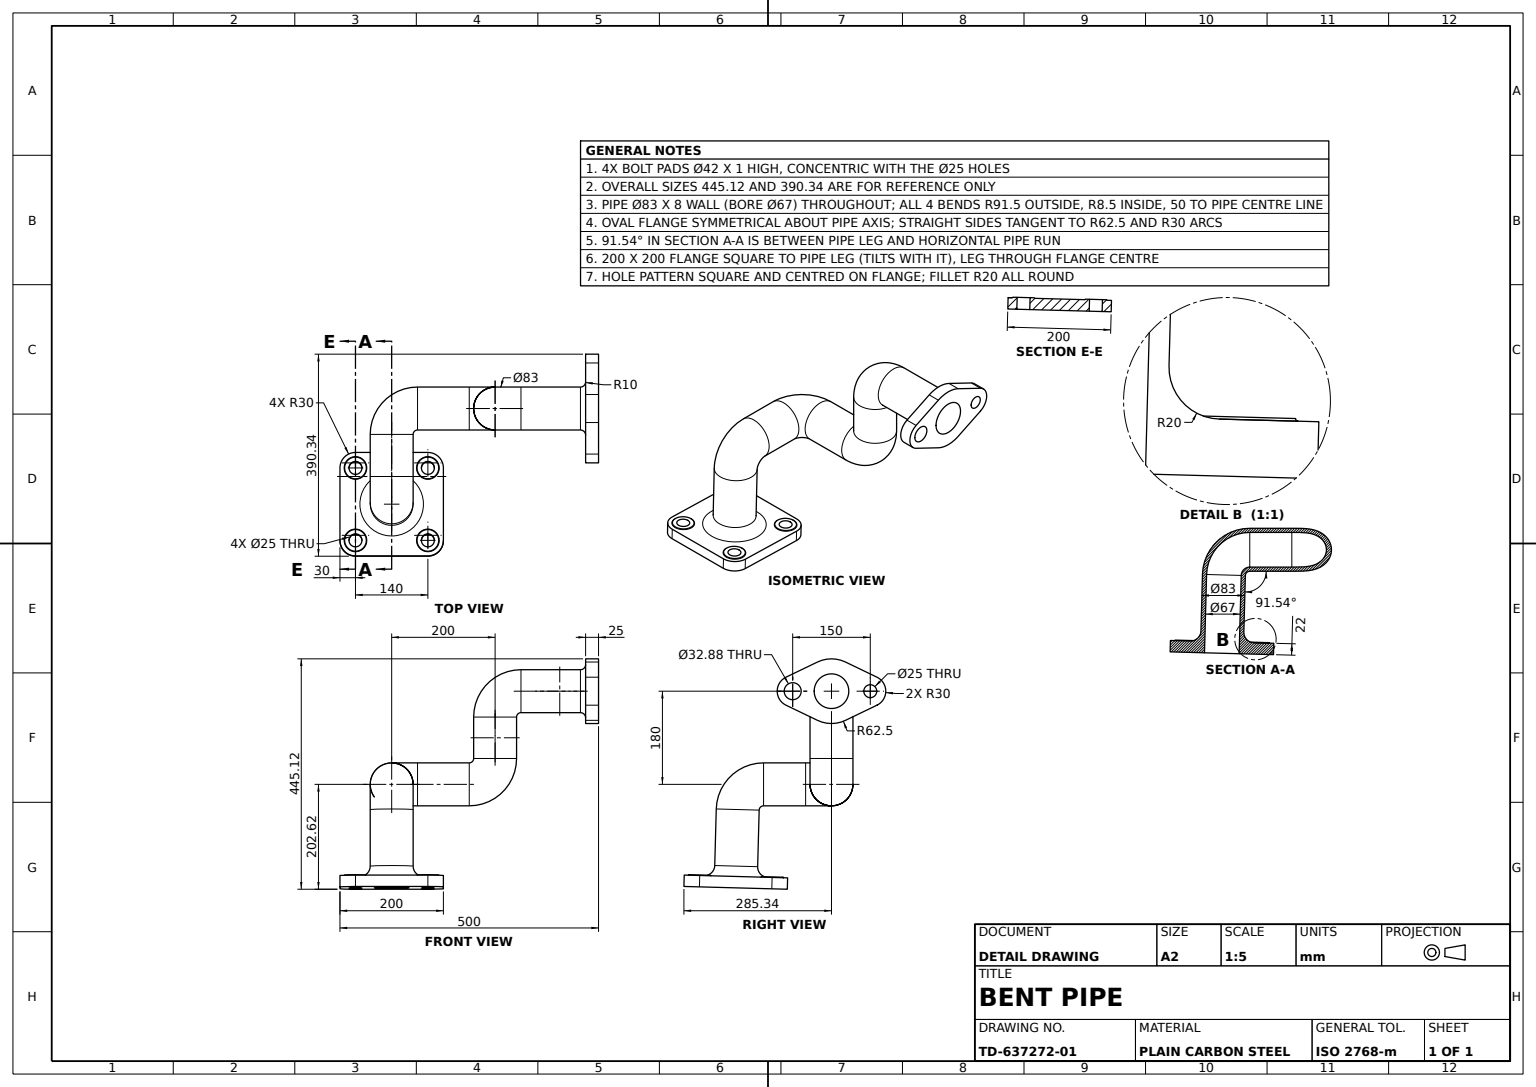
solid
v1 (0,0,-105)
v2 (0,27.037012,-88)
e1 v1 v2 CIRCLE(AX(P(0,0,-75),D(1,0,0),D(0,0,-1)),30)
v3 (-25,0,-105)
e2 v3 v1 LINE
v4 (-25,27.037012,-88)
e3 v3 v4 CIRCLE(AX(P(-25,0,-75),D(1,0,0),D(0,0,-1)),30)
e4 v4 v2 LINE
face CYL(AX(P(-25,0,-75),D(1,0,0),D(0,0,-1)),30) [-e1 -e2 e3 e4]
v5 (-25,0,-62.5)
v6 (-25,0,-87.5)
e5 v5 v6 CIRCLE(AX(P(-25,0,-75),D(1,0,0),D(0,0,-1)),12.5)
e6 v6 v5 CIRCLE(AX(P(-25,0,-75),D(1,0,0),D(0,0,-1)),12.5)
v7 (-25,27.037012,88)
v8 (-25,-27.037012,88)
e7 v7 v8 CIRCLE(AX(P(-25,0,75),D(1,0,0),D(0,0,-1)),30)
v9 (-25,56.327108,27.083333)
e8 v9 v7 LINE
v10 (-25,56.327108,-27.083333)
e9 v10 v9 CIRCLE(AX(P(-25,0,0),D(1,0,0),D(0,0,-1)),62.5)
e10 v4 v10 LINE
v11 (-25,-27.037012,-88)
e11 v11 v3 CIRCLE(AX(P(-25,0,-75),D(1,0,0),D(0,0,-1)),30)
v12 (-25,-56.327108,-27.083333)
e12 v12 v11 LINE
v13 (-25,-56.327108,27.083333)
e13 v13 v12 CIRCLE(AX(P(-25,0,0),D(1,0,0),D(0,0,-1)),62.5)
e14 v8 v13 LINE
v14 (-25,0,-51.5)
v15 (-25,0,51.5)
e15 v14 v15 CIRCLE(AX(P(-25,0,0),D(1,0,0),D(0,0,-1)),51.5)
e16 v15 v14 CIRCLE(AX(P(-25,0,0),D(1,0,0),D(0,0,-1)),51.5)
v16 (-25,0,91.441402)
v17 (-25,0,58.558598)
e17 v16 v17 CIRCLE(AX(P(-25,0,75),D(1,0,0),D(0,0,-1)),16.441402)
e18 v17 v16 CIRCLE(AX(P(-25,0,75),D(1,0,0),D(0,0,-1)),16.441402)
face PLANE(AX(P(-25,0,75),D(1,0,0),D(0,0,-1))) rev [e5 e6] [-e7 -e8 -e9 -e10 -e3 -e11 -e12 -e13 -e14] [e15 e16] [e17 e18]
v18 (0,-27.037012,88)
e19 v8 v18 LINE
v19 (0,27.037012,88)
e20 v19 v18 CIRCLE(AX(P(0,0,75),D(1,0,0),D(0,0,-1)),30)
e21 v7 v19 LINE
face CYL(AX(P(-25,0,75),D(1,0,0),D(0,0,-1)),30) [e7 e19 -e20 -e21]
v20 (-330,-355.247197,284.74932)
v21 (-330,-377.239245,285.340782)
e22 v20 v21 LINE
v22 (-300,-378.045784,255.351625)
e23 v22 v21 CIRCLE(AX(P(-330,-378.045784,255.351625),D(0,-0.999638543,0.026884636),D(0,-0.026884636,-0.999638543)),30)
v23 (-300,-356.053736,254.760163)
e24 v23 v22 LINE
e25 v23 v20 CIRCLE(AX(P(-330,-356.053736,254.760163),D(0,-0.999638543,0.026884636),D(0,-0.026884636,-0.999638543)),30)
face CYL(AX(P(-330,-356.053736,254.760163),D(0,-0.999638543,0.026884636),D(0,-0.026884636,-0.999638543)),30) [e22 -e23 -e24 e25]
v24 (0,-56.327108,27.083333)
e26 v13 v24 LINE
v25 (0,-56.327108,-27.083333)
e27 v12 v25 LINE
e28 v24 v25 CIRCLE(AX(P(0,0,0),D(1,0,0),D(0,0,-1)),62.5)
face CYL(AX(P(-25,0,0),D(1,0,0),D(0,0,-1)),62.5) [-e26 e13 e27 -e28]
v26 (-200,-50,-33.5)
v27 (-200,-130,-33.5)
e29 v26 v27 LINE
v28 (-233.5,-50,0)
e30 v26 v28 CIRCLE(AX(P(-200,-50,0),D(0,1,0),D(-1,0,0)),33.5)
v29 (-200,-50,33.5)
e31 v28 v29 CIRCLE(AX(P(-200,-50,0),D(0,1,0),D(-1,0,0)),33.5)
v30 (-200,-130,33.5)
e32 v29 v30 LINE
v31 (-233.5,-130,0)
e33 v31 v30 CIRCLE(AX(P(-200,-130,0),D(0,1,0),D(0,0,-1)),33.5)
e34 v27 v31 CIRCLE(AX(P(-200,-130,0),D(0,1,0),D(0,0,-1)),33.5)
face CYL(AX(P(-200,-50,0),D(0,-1,0),D(0,0,-1)),33.5) rev [-e29 e30 e31 e32 -e33 -e34]
v32 (-500,-359.817585,114.810767)
v33 (-500,-381.809633,115.402229)
e35 v32 v33 LINE
v34 (-470,-360.624124,84.821611)
e36 v32 v34 CIRCLE(AX(P(-470,-359.817585,114.810767),D(0,-0.999638543,0.026884636),D(0,-0.026884636,-0.999638543)),30)
v35 (-470,-382.616172,85.413073)
e37 v34 v35 LINE
e38 v33 v35 CIRCLE(AX(P(-470,-381.809633,115.402229),D(0,-0.999638543,0.026884636),D(0,-0.026884636,-0.999638543)),30)
face CYL(AX(P(-470,-359.817585,114.810767),D(0,-0.999638543,0.026884636),D(0,-0.026884636,-0.999638543)),30) [-e35 e36 e37 -e38]
v36 (-470,-378.381842,242.856143)
v37 (-470,-377.709726,267.847107)
e39 v36 v37 CIRCLE(AX(P(-470,-378.045784,255.351625),D(0,-0.999638543,0.026884636),D(0,-0.026884636,-0.999638543)),12.5)
v38 (-470,-354.71804,267.22876)
e40 v38 v37 LINE
v39 (-470,-355.390155,242.237797)
e41 v38 v39 CIRCLE(AX(P(-470,-355.054098,254.733279),D(0,0.999638543,-0.026884636),D(0,0.026884636,0.999638543)),12.5)
e42 v39 v36 LINE
face CYL(AX(P(-470,-356.053736,254.760163),D(0,-0.999638543,0.026884636),D(0,-0.026884636,-0.999638543)),12.5) rev [e39 -e40 e41 e42]
v40 (-330,-381.473575,127.897711)
v41 (-330,-382.145691,102.906747)
e43 v40 v41 CIRCLE(AX(P(-330,-381.809633,115.402229),D(0,-0.999638543,0.026884636),D(0,-0.026884636,-0.999638543)),12.5)
v42 (-330,-359.154005,102.288401)
e44 v42 v41 LINE
v43 (-330,-358.481889,127.279364)
e45 v42 v43 CIRCLE(AX(P(-330,-358.817947,114.783883),D(0,0.999638543,-0.026884636),D(0,0.026884636,0.999638543)),12.5)
e46 v43 v40 LINE
face CYL(AX(P(-330,-359.817585,114.810767),D(0,-0.999638543,0.026884636),D(0,-0.026884636,-0.999638543)),12.5) rev [e43 -e44 e45 e46]
v44 (-350,-213.5,0)
v45 (-350,-180,-33.5)
e47 v44 v45 CIRCLE(AX(P(-350,-180,0),D(1,0,0),D(0,-1,0)),33.5)
v46 (-250,-213.5,0)
e48 v46 v44 LINE
v47 (-250,-146.5,0)
e49 v46 v47 CIRCLE(AX(P(-250,-180,0),D(1,0,0),D(0,1,0)),33.5)
v48 (-350,-146.5,0)
e50 v47 v48 LINE
e51 v45 v48 CIRCLE(AX(P(-350,-180,0),D(1,0,0),D(0,-1,0)),33.5)
face CYL(AX(P(-250,-180,0),D(-1,0,0),D(0,-1,0)),33.5) rev [-e47 -e48 e49 e50 -e51]
v49 (0,0,58.558598)
v50 (0,0,91.441402)
e52 v49 v50 CIRCLE(AX(P(0,0,75),D(1,0,0),D(0,0,-1)),16.441402)
e53 v16 v50 LINE
e54 v17 v49 LINE
face CYL(AX(P(-25,0,75),D(1,0,0),D(0,0,-1)),16.441402) rev [e52 -e53 -e18 e54]
v51 (-433.5,-180,50)
v52 (-366.5,-180,50)
e55 v51 v52 CIRCLE(AX(P(-400,-180,50),D(0,0,-1),D(-1,0,0)),33.5)
e56 v45 v51 CIRCLE(AX(P(-350,-180,50),D(0,1,0),D(0,0,1)),83.5)
v53 (-350,-180,33.5)
e57 v48 v53 CIRCLE(AX(P(-350,-180,0),D(1,0,0),D(0,-1,0)),33.5)
e58 v53 v52 CIRCLE(AX(P(-350,-180,50),D(0,1,0),D(0,0,1)),16.5)
face TORUS(AX(P(-350,-180,50),D(0,1,0),D(0,0,1)),50,33.5) rev [-e55 -e56 e51 e57 e58]
v54 (-500,-378.045784,255.351625)
e59 v54 v33 LINE
v55 (-500,-356.053736,254.760163)
e60 v55 v54 LINE
e61 v55 v32 LINE
face PLANE(AX(P(-500,-359.817585,114.810767),D(-1,0,0),D(0,-1,0))) [-e59 -e60 e61 e35]
v56 (-330,-355.462274,276.752211)
v57 (-330,-356.645198,232.768115)
e62 v56 v57 CIRCLE(AX(P(-330,-356.053736,254.760163),D(0,-0.999638543,0.026884636),D(0,-0.026884636,-0.999638543)),22)
v58 (-330,-354.48952,275.725688)
e63 v56 v58 CIRCLE(AX(P(-330,-354.462636,276.725327),D(1,0,0),D(0,1,0)),1)
v59 (-330,-355.618675,233.740869)
e64 v59 v58 CIRCLE(AX(P(-330,-355.054098,254.733279),D(0,0.999638543,-0.026884636),D(0,0.026884636,0.999638543)),21)
e65 v57 v59 CIRCLE(AX(P(-330,-355.64556,232.741231),D(-1,0,0),D(0,-1,0)),1)
face TORUS(AX(P(-330,-355.054098,254.733279),D(0,-0.999638543,0.026884636),D(0,-0.026884636,-0.999638543)),22,1) rev [-e62 e63 -e64 -e65]
v60 (-400,-138.5,131.326638)
v61 (-358.5,-180,131.326638)
e66 v60 v61 CIRCLE(AX(P(-400,-180,131.326638),D(0,0,-1),D(1,0,0)),41.5)
v62 (-358.5,-180,50)
e67 v62 v61 LINE
v63 (-441.5,-180,50)
e68 v63 v62 CIRCLE(AX(P(-400,-180,50),D(0,0,-1),D(-1,0,0)),41.5)
v64 (-441.5,-180,131.326638)
e69 v63 v64 LINE
e70 v64 v60 CIRCLE(AX(P(-400,-180,131.326638),D(0,0,-1),D(1,0,0)),41.5)
face CYL(AX(P(-400,-180,50),D(0,0,1),D(1,0,0)),41.5) [e66 -e67 -e68 e69 e70]
e71 v58 v59 CIRCLE(AX(P(-330,-355.054098,254.733279),D(0,0.999638543,-0.026884636),D(0,0.026884636,0.999638543)),21)
e72 v57 v56 CIRCLE(AX(P(-330,-356.053736,254.760163),D(0,-0.999638543,0.026884636),D(0,-0.026884636,-0.999638543)),22)
face TORUS(AX(P(-330,-355.054098,254.733279),D(0,-0.999638543,0.026884636),D(0,-0.026884636,-0.999638543)),22,1) rev [e65 -e71 -e63 -e72]
v65 (-150,0,41.5)
v66 (-150,-41.5,0)
e73 v65 v66 CIRCLE(AX(P(-150,0,0),D(1,0,0),D(0,0,1)),41.5)
v67 (-150,41.5,0)
e74 v67 v65 CIRCLE(AX(P(-150,0,0),D(1,0,0),D(0,0,1)),41.5)
v68 (-241.5,-50,0)
e75 v67 v68 CIRCLE(AX(P(-150,-50,0),D(0,0,1),D(0,-1,0)),91.5)
v69 (-200,-50,41.5)
e76 v68 v69 CIRCLE(AX(P(-200,-50,0),D(0,1,0),D(-1,0,0)),41.5)
v70 (-158.5,-50,0)
e77 v69 v70 CIRCLE(AX(P(-200,-50,0),D(0,1,0),D(-1,0,0)),41.5)
e78 v66 v70 CIRCLE(AX(P(-150,-50,0),D(0,0,1),D(0,-1,0)),8.5)
face TORUS(AX(P(-150,-50,0),D(0,0,1),D(0,-1,0)),50,41.5) [-e73 -e74 e75 e76 e77 -e78]
v71 (-150,-33.5,0)
v72 (-150,0,-33.5)
e79 v71 v72 CIRCLE(AX(P(-150,0,0),D(1,0,0),D(0,0,1)),33.5)
v73 (-150,0,33.5)
e80 v73 v71 CIRCLE(AX(P(-150,0,0),D(1,0,0),D(0,0,1)),33.5)
v74 (0,0,33.5)
e81 v74 v73 LINE
v75 (0,0,-33.5)
e82 v74 v75 CIRCLE(AX(P(0,0,0),D(1,0,0),D(0,0,-1)),33.5)
e83 v75 v72 LINE
face CYL(AX(P(0,0,0),D(-1,0,0),D(0,0,1)),33.5) rev [-e79 -e80 -e81 e82 e83]
v76 (-433.5,-180,131.326638)
e84 v51 v76 LINE
v77 (-400,-213.5,131.326638)
e85 v77 v76 CIRCLE(AX(P(-400,-180,131.326638),D(0,0,-1),D(1,0,0)),33.5)
v78 (-366.5,-180,131.326638)
e86 v78 v77 CIRCLE(AX(P(-400,-180,131.326638),D(0,0,-1),D(1,0,0)),33.5)
e87 v52 v78 LINE
e88 v52 v51 CIRCLE(AX(P(-400,-180,50),D(0,0,-1),D(-1,0,0)),33.5)
face CYL(AX(P(-400,-180,50),D(0,0,1),D(1,0,0)),33.5) rev [e84 -e85 -e86 -e87 e88]
v79 (-470,-355.462274,276.752211)
v80 (-470,-354.48952,275.725688)
e89 v79 v80 CIRCLE(AX(P(-470,-354.462636,276.725327),D(1,0,0),D(0,1,0)),1)
v81 (-470,-355.618675,233.740869)
e90 v81 v80 CIRCLE(AX(P(-470,-355.054098,254.733279),D(0,0.999638543,-0.026884636),D(0,0.026884636,0.999638543)),21)
v82 (-470,-356.645198,232.768115)
e91 v82 v81 CIRCLE(AX(P(-470,-355.64556,232.741231),D(-1,0,0),D(0,-1,0)),1)
e92 v79 v82 CIRCLE(AX(P(-470,-356.053736,254.760163),D(0,-0.999638543,0.026884636),D(0,-0.026884636,-0.999638543)),22)
face TORUS(AX(P(-470,-355.054098,254.733279),D(0,-0.999638543,0.026884636),D(0,-0.026884636,-0.999638543)),22,1) rev [e89 -e90 -e91 -e92]
v83 (-330,-354.71804,267.22876)
v84 (-330,-355.390155,242.237797)
e93 v83 v84 CIRCLE(AX(P(-330,-355.054098,254.733279),D(0,0.999638543,-0.026884636),D(0,0.026884636,0.999638543)),12.5)
e94 v84 v83 CIRCLE(AX(P(-330,-355.054098,254.733279),D(0,0.999638543,-0.026884636),D(0,0.026884636,0.999638543)),12.5)
face PLANE(AX(P(-330,-355.054098,254.733279),D(0,0.999638543,-0.026884636),D(0,0.026884636,0.999638543))) [-e93 -e94] [e64 e71]
e95 v31 v47 CIRCLE(AX(P(-250,-130,0),D(0,0,-1),D(-1,0,0)),16.5)
v85 (-166.5,-130,0)
e96 v30 v85 CIRCLE(AX(P(-200,-130,0),D(0,1,0),D(0,0,-1)),33.5)
e97 v85 v46 CIRCLE(AX(P(-250,-130,0),D(0,0,-1),D(-1,0,0)),83.5)
e98 v47 v46 CIRCLE(AX(P(-250,-180,0),D(1,0,0),D(0,1,0)),33.5)
face TORUS(AX(P(-250,-130,0),D(0,0,-1),D(-1,0,0)),50,33.5) rev [-e95 e33 e96 e97 -e98]
e99 v53 v44 CIRCLE(AX(P(-350,-180,0),D(1,0,0),D(0,-1,0)),33.5)
face TORUS(AX(P(-350,-180,50),D(0,1,0),D(0,0,1)),50,33.5) rev [e56 -e88 -e58 e99 e47]
e100 v85 v27 CIRCLE(AX(P(-200,-130,0),D(0,1,0),D(0,0,-1)),33.5)
face TORUS(AX(P(-250,-130,0),D(0,0,-1),D(-1,0,0)),50,33.5) rev [e100 e34 e95 -e49 -e97]
v86 (-470,-359.226123,136.802815)
v87 (-470,-358.253369,135.776292)
e101 v86 v87 CIRCLE(AX(P(-470,-358.226485,136.775931),D(1,0,0),D(0,1,0)),1)
v88 (-470,-359.382524,93.791473)
e102 v88 v87 CIRCLE(AX(P(-470,-358.817947,114.783883),D(0,0.999638543,-0.026884636),D(0,0.026884636,0.999638543)),21)
v89 (-470,-360.409047,92.818719)
e103 v89 v88 CIRCLE(AX(P(-470,-359.409409,92.791835),D(-1,0,0),D(0,-1,0)),1)
e104 v86 v89 CIRCLE(AX(P(-470,-359.817585,114.810767),D(0,-0.999638543,0.026884636),D(0,-0.026884636,-0.999638543)),22)
face TORUS(AX(P(-470,-358.817947,114.783883),D(0,-0.999638543,0.026884636),D(0,-0.026884636,-0.999638543)),22,1) rev [e101 -e102 -e103 -e104]
v90 (0,0,-87.5)
v91 (0,0,-62.5)
e105 v90 v91 CIRCLE(AX(P(0,0,-75),D(1,0,0),D(0,0,-1)),12.5)
e106 v91 v90 CIRCLE(AX(P(0,0,-75),D(1,0,0),D(0,0,-1)),12.5)
e107 v18 v24 LINE
v92 (0,-27.037012,-88)
e108 v25 v92 LINE
e109 v92 v1 CIRCLE(AX(P(0,0,-75),D(1,0,0),D(0,0,-1)),30)
v93 (0,56.327108,-27.083333)
e110 v2 v93 LINE
v94 (0,56.327108,27.083333)
e111 v93 v94 CIRCLE(AX(P(0,0,0),D(1,0,0),D(0,0,-1)),62.5)
e112 v94 v19 LINE
e113 v75 v74 CIRCLE(AX(P(0,0,0),D(1,0,0),D(0,0,-1)),33.5)
e114 v50 v49 CIRCLE(AX(P(0,0,75),D(1,0,0),D(0,0,-1)),16.441402)
face PLANE(AX(P(0,0,0),D(1,0,0),D(0,1,0))) [-e105 -e106] [e20 e107 e28 e108 e109 e1 e110 e111 e112] [-e113 -e82] [-e114 -e52]
v95 (-400,-380.828344,151.889036)
v96 (-400,-379.027073,218.864818)
e115 v95 v96 CIRCLE(AX(P(-400,-379.927709,185.376927),D(0,0.999638543,-0.026884636),D(0,0.026884636,0.999638543)),33.5)
v97 (-400,-229.556404,147.820674)
e116 v97 v95 LINE
v98 (-400,-227.755133,214.796457)
e117 v97 v98 CIRCLE(AX(P(-400,-228.655768,181.308566),D(0,0.999638543,-0.026884636),D(0,0.026884636,0.999638543)),33.5)
e118 v98 v96 LINE
face CYL(AX(P(-400,-228.655768,181.308566),D(0,-0.999638543,0.026884636),D(0,-0.026884636,-0.999638543)),33.5) rev [-e115 -e116 e117 e118]
v99 (-150,0,-41.5)
e119 v99 v67 CIRCLE(AX(P(-150,0,0),D(1,0,0),D(0,0,1)),41.5)
e120 v66 v99 CIRCLE(AX(P(-150,0,0),D(1,0,0),D(0,0,1)),41.5)
v100 (-200,-50,-41.5)
e121 v70 v100 CIRCLE(AX(P(-200,-50,0),D(0,1,0),D(-1,0,0)),41.5)
e122 v100 v68 CIRCLE(AX(P(-200,-50,0),D(0,1,0),D(-1,0,0)),41.5)
face TORUS(AX(P(-150,-50,0),D(0,0,1),D(0,-1,0)),50,41.5) [-e119 -e120 e78 e121 e122 -e75]
v101 (-158.5,-130,0)
v102 (-200,-130,-41.5)
e123 v101 v102 CIRCLE(AX(P(-200,-130,0),D(0,1,0),D(0,0,-1)),41.5)
v103 (-250,-221.5,0)
e124 v101 v103 CIRCLE(AX(P(-250,-130,0),D(0,0,-1),D(-1,0,0)),91.5)
v104 (-250,-138.5,0)
e125 v103 v104 CIRCLE(AX(P(-250,-180,0),D(1,0,0),D(0,1,0)),41.5)
v105 (-241.5,-130,0)
e126 v105 v104 CIRCLE(AX(P(-250,-130,0),D(0,0,-1),D(-1,0,0)),8.5)
e127 v102 v105 CIRCLE(AX(P(-200,-130,0),D(0,1,0),D(0,0,-1)),41.5)
face TORUS(AX(P(-250,-130,0),D(0,0,-1),D(-1,0,0)),50,41.5) [-e123 e124 e125 -e126 -e127]
v106 (-400,-229.771481,139.823566)
v107 (-400,-227.540056,222.793565)
e128 v106 v107 CIRCLE(AX(P(-400,-228.655768,181.308566),D(0,0.999638543,-0.026884636),D(0,0.026884636,0.999638543)),41.5)
v108 (-400,-339.058602,142.762773)
e129 v106 v108 LINE
v109 (-400,-336.827177,225.732772)
e130 v108 v109 CIRCLE(AX(P(-400,-337.94289,184.247773),D(0,0.999638543,-0.026884636),D(0,-0.026884636,-0.999638543)),41.5)
e131 v107 v109 LINE
face CYL(AX(P(-400,-228.655768,181.308566),D(0,-0.999638543,0.026884636),D(0,-0.026884636,-0.999638543)),41.5) [-e128 e129 e130 -e131]
v110 (-400,-221.5,131.326638)
e132 v110 v64 CIRCLE(AX(P(-400,-180,131.326638),D(0,0,-1),D(1,0,0)),41.5)
e133 v62 v63 CIRCLE(AX(P(-400,-180,50),D(0,0,-1),D(-1,0,0)),41.5)
e134 v61 v110 CIRCLE(AX(P(-400,-180,131.326638),D(0,0,-1),D(1,0,0)),41.5)
face CYL(AX(P(-400,-180,50),D(0,0,1),D(1,0,0)),41.5) [e132 -e69 -e133 e67 e134]
v111 (-150,33.5,0)
e135 v72 v111 CIRCLE(AX(P(-150,0,0),D(1,0,0),D(0,0,1)),33.5)
e136 v111 v73 CIRCLE(AX(P(-150,0,0),D(1,0,0),D(0,0,1)),33.5)
face CYL(AX(P(0,0,0),D(-1,0,0),D(0,0,1)),33.5) rev [-e135 -e83 e113 e81 -e136]
e137 v107 v106 CIRCLE(AX(P(-400,-228.655768,181.308566),D(0,0.999638543,-0.026884636),D(0,0.026884636,0.999638543)),41.5)
e138 v109 v108 CIRCLE(AX(P(-400,-337.94289,184.247773),D(0,0.999638543,-0.026884636),D(0,-0.026884636,-0.999638543)),41.5)
face CYL(AX(P(-400,-228.655768,181.308566),D(0,-0.999638543,0.026884636),D(0,-0.026884636,-0.999638543)),41.5) [-e129 -e137 e131 e138]
e139 v82 v79 CIRCLE(AX(P(-470,-356.053736,254.760163),D(0,-0.999638543,0.026884636),D(0,-0.026884636,-0.999638543)),22)
e140 v80 v81 CIRCLE(AX(P(-470,-355.054098,254.733279),D(0,0.999638543,-0.026884636),D(0,0.026884636,0.999638543)),21)
face TORUS(AX(P(-470,-355.054098,254.733279),D(0,-0.999638543,0.026884636),D(0,-0.026884636,-0.999638543)),22,1) rev [-e139 e91 -e140 -e89]
v112 (-330,-359.226123,136.802815)
v113 (-330,-360.409047,92.818719)
e141 v112 v113 CIRCLE(AX(P(-330,-359.817585,114.810767),D(0,-0.999638543,0.026884636),D(0,-0.026884636,-0.999638543)),22)
v114 (-330,-358.253369,135.776292)
e142 v112 v114 CIRCLE(AX(P(-330,-358.226485,136.775931),D(1,0,0),D(0,1,0)),1)
v115 (-330,-359.382524,93.791473)
e143 v115 v114 CIRCLE(AX(P(-330,-358.817947,114.783883),D(0,0.999638543,-0.026884636),D(0,0.026884636,0.999638543)),21)
e144 v113 v115 CIRCLE(AX(P(-330,-359.409409,92.791835),D(-1,0,0),D(0,-1,0)),1)
face TORUS(AX(P(-330,-358.817947,114.783883),D(0,-0.999638543,0.026884636),D(0,-0.026884636,-0.999638543)),22,1) rev [-e141 e142 -e143 -e144]
v116 (-200,-130,41.5)
e145 v69 v116 LINE
e146 v100 v102 LINE
e147 v105 v116 CIRCLE(AX(P(-200,-130,0),D(0,1,0),D(0,0,-1)),41.5)
face CYL(AX(P(-200,-50,0),D(0,-1,0),D(0,0,-1)),41.5) [-e145 -e76 -e122 e146 e127 e147]
e148 v98 v97 CIRCLE(AX(P(-400,-228.655768,181.308566),D(0,0.999638543,-0.026884636),D(0,0.026884636,0.999638543)),33.5)
e149 v96 v95 CIRCLE(AX(P(-400,-379.927709,185.376927),D(0,0.999638543,-0.026884636),D(0,0.026884636,0.999638543)),33.5)
face CYL(AX(P(-400,-228.655768,181.308566),D(0,-0.999638543,0.026884636),D(0,-0.026884636,-0.999638543)),33.5) rev [-e118 e148 e116 -e149]
v117 (-35,0,41.5)
e150 v117 v65 LINE
v118 (-35,0,-41.5)
e151 v117 v118 CIRCLE(AX(P(-35,0,0),D(-1,0,0),D(0,0,-1)),41.5)
e152 v118 v99 LINE
face CYL(AX(P(0,0,0),D(-1,0,0),D(0,0,1)),41.5) [e74 -e150 e151 e152 e119]
e153 v11 v92 LINE
face CYL(AX(P(-25,0,-75),D(1,0,0),D(0,0,-1)),30) [-e153 e11 e2 -e109]
v119 (-400,-146.5,131.326638)
e154 v76 v119 CIRCLE(AX(P(-400,-180,131.326638),D(0,0,-1),D(1,0,0)),33.5)
e155 v119 v98 CIRCLE(AX(P(-400,-230,131.326638),D(1,0,0),D(0,0,-1)),83.5)
e156 v77 v97 CIRCLE(AX(P(-400,-230,131.326638),D(1,0,0),D(0,0,-1)),16.5)
face TORUS(AX(P(-400,-230,131.326638),D(1,0,0),D(0,0,-1)),50,33.5) rev [e154 e155 -e117 -e156 e85]
e157 v14 v118 CIRCLE(AX(P(-35,0,-51.5),D(0,-1,0),D(1,0,0)),10)
e158 v15 v117 CIRCLE(AX(P(-35,0,51.5),D(0,1,0),D(-1,0,0)),10)
face TORUS(AX(P(-35,0,0),D(1,0,0),D(0,0,-1)),51.5,10) rev [e157 -e151 -e158 -e15]
e159 v119 v78 CIRCLE(AX(P(-400,-180,131.326638),D(0,0,-1),D(1,0,0)),33.5)
face CYL(AX(P(-400,-180,50),D(0,0,1),D(1,0,0)),33.5) rev [-e84 e55 e87 -e159 -e154]
v120 (-470,-377.239245,285.340782)
e160 v21 v120 LINE
v121 (-470,-355.247197,284.74932)
e161 v20 v121 LINE
e162 v121 v120 LINE
face PLANE(AX(P(-470,-355.247197,284.74932),D(0,0.026884636,0.999638543),D(0,-0.999638543,0.026884636))) [-e160 -e22 e161 e162]
e163 v43 v42 CIRCLE(AX(P(-330,-358.817947,114.783883),D(0,0.999638543,-0.026884636),D(0,0.026884636,0.999638543)),12.5)
e164 v114 v115 CIRCLE(AX(P(-330,-358.817947,114.783883),D(0,0.999638543,-0.026884636),D(0,0.026884636,0.999638543)),21)
face PLANE(AX(P(-330,-358.817947,114.783883),D(0,0.999638543,-0.026884636),D(0,0.026884636,0.999638543))) [-e163 -e45] [e143 e164]
e165 v5 v91 LINE
e166 v6 v90 LINE
face CYL(AX(P(-25,0,-75),D(1,0,0),D(0,0,-1)),12.5) rev [-e5 e165 e106 -e166]
e167 v10 v93 LINE
face PLANE(AX(P(-25,27.037012,-88),D(0,0.901233722,-0.433333333),D(0,0.433333333,0.901233722))) [-e110 -e4 e10 e167]
e168 v39 v38 CIRCLE(AX(P(-470,-355.054098,254.733279),D(0,0.999638543,-0.026884636),D(0,0.026884636,0.999638543)),12.5)
face PLANE(AX(P(-470,-355.054098,254.733279),D(0,0.999638543,-0.026884636),D(0,0.026884636,0.999638543))) [-e41 -e168] [e90 e140]
e169 v116 v101 CIRCLE(AX(P(-200,-130,0),D(0,1,0),D(0,0,-1)),41.5)
e170 v104 v103 CIRCLE(AX(P(-250,-180,0),D(1,0,0),D(0,1,0)),41.5)
face TORUS(AX(P(-250,-130,0),D(0,0,-1),D(-1,0,0)),50,41.5) [-e124 -e169 -e147 e126 e170]
v122 (-350,-221.5,0)
e171 v103 v122 LINE
v123 (-350,-138.5,0)
e172 v104 v123 LINE
v124 (-350,-180,41.5)
e173 v123 v124 CIRCLE(AX(P(-350,-180,0),D(1,0,0),D(0,-1,0)),41.5)
e174 v124 v122 CIRCLE(AX(P(-350,-180,0),D(1,0,0),D(0,-1,0)),41.5)
face CYL(AX(P(-250,-180,0),D(-1,0,0),D(0,-1,0)),41.5) [-e171 -e170 e172 e173 e174]
face CYL(AX(P(-200,-50,0),D(0,-1,0),D(0,0,-1)),41.5) [e145 e169 e123 -e146 -e121 -e77]
e175 v41 v40 CIRCLE(AX(P(-330,-381.809633,115.402229),D(0,-0.999638543,0.026884636),D(0,-0.026884636,-0.999638543)),12.5)
face CYL(AX(P(-330,-359.817585,114.810767),D(0,-0.999638543,0.026884636),D(0,-0.026884636,-0.999638543)),12.5) rev [-e46 e163 e44 e175]
e176 v89 v86 CIRCLE(AX(P(-470,-359.817585,114.810767),D(0,-0.999638543,0.026884636),D(0,-0.026884636,-0.999638543)),22)
v125 (-400,-359.589066,123.307695)
v126 (-400,-356.282255,246.263236)
e177 v125 v126 CIRCLE(AX(P(-400,-357.935661,184.785465),D(0,-0.999638543,0.026884636),D(0,-0.026884636,-0.999638543)),61.5)
e178 v126 v125 CIRCLE(AX(P(-400,-357.935661,184.785465),D(0,-0.999638543,0.026884636),D(0,-0.026884636,-0.999638543)),61.5)
e179 v121 v55 CIRCLE(AX(P(-470,-356.053736,254.760163),D(0,-0.999638543,0.026884636),D(0,-0.026884636,-0.999638543)),30)
v127 (-300,-359.817585,114.810767)
e180 v127 v23 LINE
v128 (-330,-360.624124,84.821611)
e181 v128 v127 CIRCLE(AX(P(-330,-359.817585,114.810767),D(0,-0.999638543,0.026884636),D(0,-0.026884636,-0.999638543)),30)
e182 v34 v128 LINE
e183 v113 v112 CIRCLE(AX(P(-330,-359.817585,114.810767),D(0,-0.999638543,0.026884636),D(0,-0.026884636,-0.999638543)),22)
face PLANE(AX(P(-470,-359.817585,114.810767),D(0,-0.999638543,0.026884636),D(0,-0.026884636,-0.999638543))) rev [e62 e72] [e92 e139] [e176 e104] [e177 e178] [-e61 -e179 -e161 -e25 -e180 -e181 -e182 -e36] [e183 e141]
face TORUS(AX(P(-400,-230,131.326638),D(1,0,0),D(0,0,-1)),50,33.5) rev [e159 e86 e156 -e148 -e155]
v129 (-300,-381.809633,115.402229)
e184 v129 v22 LINE
e185 v120 v54 CIRCLE(AX(P(-470,-378.045784,255.351625),D(0,-0.999638543,0.026884636),D(0,-0.026884636,-0.999638543)),30)
v130 (-330,-382.616172,85.413073)
e186 v35 v130 LINE
e187 v130 v129 CIRCLE(AX(P(-330,-381.809633,115.402229),D(0,-0.999638543,0.026884636),D(0,-0.026884636,-0.999638543)),30)
v131 (-470,-381.473575,127.897711)
v132 (-470,-382.145691,102.906747)
e188 v131 v132 CIRCLE(AX(P(-470,-381.809633,115.402229),D(0,-0.999638543,0.026884636),D(0,-0.026884636,-0.999638543)),12.5)
e189 v132 v131 CIRCLE(AX(P(-470,-381.809633,115.402229),D(0,-0.999638543,0.026884636),D(0,-0.026884636,-0.999638543)),12.5)
v133 (-330,-378.381842,242.856143)
v134 (-330,-377.709726,267.847107)
e190 v133 v134 CIRCLE(AX(P(-330,-378.045784,255.351625),D(0,-0.999638543,0.026884636),D(0,-0.026884636,-0.999638543)),12.5)
e191 v134 v133 CIRCLE(AX(P(-330,-378.045784,255.351625),D(0,-0.999638543,0.026884636),D(0,-0.026884636,-0.999638543)),12.5)
e192 v37 v36 CIRCLE(AX(P(-470,-378.045784,255.351625),D(0,-0.999638543,0.026884636),D(0,-0.026884636,-0.999638543)),12.5)
face PLANE(AX(P(-400,-379.927709,185.376927),D(0,0.999638543,-0.026884636),D(0,0.026884636,0.999638543))) rev [e184 e23 e160 e185 e59 e38 e186 e187] [-e188 -e189] [e149 e115] [-e190 -e191] [-e39 -e192] [-e43 -e175]
e193 v127 v129 LINE
face PLANE(AX(P(-300,-359.817585,114.810767),D(1,0,0),D(0,1,0))) [-e184 -e193 e180 e24]
v135 (-350,-180,-41.5)
e194 v122 v135 CIRCLE(AX(P(-350,-180,0),D(1,0,0),D(0,-1,0)),41.5)
e195 v124 v62 CIRCLE(AX(P(-350,-180,50),D(0,1,0),D(0,0,1)),8.5)
e196 v135 v63 CIRCLE(AX(P(-350,-180,50),D(0,1,0),D(0,0,1)),91.5)
face TORUS(AX(P(-350,-180,50),D(0,1,0),D(0,0,1)),50,41.5) [-e194 -e174 e195 e133 -e196]
v136 (-470,-358.481889,127.279364)
e197 v136 v131 LINE
v137 (-470,-359.154005,102.288401)
e198 v136 v137 CIRCLE(AX(P(-470,-358.817947,114.783883),D(0,0.999638543,-0.026884636),D(0,0.026884636,0.999638543)),12.5)
e199 v137 v132 LINE
face CYL(AX(P(-470,-359.817585,114.810767),D(0,-0.999638543,0.026884636),D(0,-0.026884636,-0.999638543)),12.5) rev [-e197 e198 e199 e189]
e200 v84 v133 LINE
e201 v83 v134 LINE
face CYL(AX(P(-330,-356.053736,254.760163),D(0,-0.999638543,0.026884636),D(0,-0.026884636,-0.999638543)),12.5) rev [e200 e190 -e201 e93]
e202 v87 v88 CIRCLE(AX(P(-470,-358.817947,114.783883),D(0,0.999638543,-0.026884636),D(0,0.026884636,0.999638543)),21)
face TORUS(AX(P(-470,-358.817947,114.783883),D(0,-0.999638543,0.026884636),D(0,-0.026884636,-0.999638543)),22,1) rev [-e176 e103 -e202 -e101]
face CYL(AX(P(-25,0,-75),D(1,0,0),D(0,0,-1)),12.5) rev [-e165 -e6 e166 e105]
e203 v118 v117 CIRCLE(AX(P(-35,0,0),D(-1,0,0),D(0,0,-1)),41.5)
face TORUS(AX(P(-35,0,0),D(1,0,0),D(0,0,-1)),51.5,10) rev [-e203 -e157 -e16 e158]
e204 v137 v136 CIRCLE(AX(P(-470,-358.817947,114.783883),D(0,0.999638543,-0.026884636),D(0,0.026884636,0.999638543)),12.5)
face CYL(AX(P(-470,-359.817585,114.810767),D(0,-0.999638543,0.026884636),D(0,-0.026884636,-0.999638543)),12.5) rev [e188 -e199 e204 e197]
e205 v128 v130 LINE
face PLANE(AX(P(-470,-360.624124,84.821611),D(0,-0.026884636,-0.999638543),D(0,0.999638543,-0.026884636))) [-e37 e182 e205 -e186]
e206 v9 v94 LINE
face PLANE(AX(P(-25,27.037012,88),D(0,0.901233722,0.433333333),D(0,-0.433333333,0.901233722))) [e8 e21 -e112 -e206]
e207 v135 v123 CIRCLE(AX(P(-350,-180,0),D(1,0,0),D(0,-1,0)),41.5)
face CYL(AX(P(-250,-180,0),D(-1,0,0),D(0,-1,0)),41.5) [-e172 -e125 e171 e194 e207]
e208 v126 v109 CIRCLE(AX(P(-400,-336.289485,245.725543),D(1,0,0),D(0,1,0)),20)
e209 v125 v108 CIRCLE(AX(P(-400,-339.596295,122.770002),D(-1,0,0),D(0,-1,0)),20)
face TORUS(AX(P(-400,-337.94289,184.247773),D(0,-0.999638543,0.026884636),D(0,-0.026884636,-0.999638543)),61.5,20) rev [-e178 e208 -e130 -e209]
face TORUS(AX(P(-350,-180,50),D(0,1,0),D(0,0,1)),50,41.5) [-e207 e196 e68 -e195 -e173]
face CYL(AX(P(-330,-356.053736,254.760163),D(0,-0.999638543,0.026884636),D(0,-0.026884636,-0.999638543)),12.5) rev [e201 e191 -e200 e94]
e210 v110 v106 CIRCLE(AX(P(-400,-230,131.326638),D(1,0,0),D(0,0,-1)),8.5)
e211 v60 v107 CIRCLE(AX(P(-400,-230,131.326638),D(1,0,0),D(0,0,-1)),91.5)
face TORUS(AX(P(-400,-230,131.326638),D(1,0,0),D(0,0,-1)),50,41.5) [e137 -e210 -e134 -e66 e211]
face CYL(AX(P(-470,-356.053736,254.760163),D(0,-0.999638543,0.026884636),D(0,-0.026884636,-0.999638543)),30) [-e162 e179 e60 -e185]
face CYL(AX(P(0,0,0),D(-1,0,0),D(0,0,1)),41.5) [-e152 e203 e150 e73 e120]
e212 v111 v28 CIRCLE(AX(P(-150,-50,0),D(0,0,1),D(0,-1,0)),83.5)
v138 (-166.5,-50,0)
e213 v138 v26 CIRCLE(AX(P(-200,-50,0),D(0,1,0),D(-1,0,0)),33.5)
e214 v71 v138 CIRCLE(AX(P(-150,-50,0),D(0,0,1),D(0,-1,0)),16.5)
face TORUS(AX(P(-150,-50,0),D(0,0,1),D(0,-1,0)),50,33.5) rev [e135 e212 -e30 -e213 -e214 e79]
face PLANE(AX(P(-470,-358.817947,114.783883),D(0,0.999638543,-0.026884636),D(0,0.026884636,0.999638543))) [-e204 -e198] [e202 e102]
face TORUS(AX(P(-400,-230,131.326638),D(1,0,0),D(0,0,-1)),50,41.5) [-e132 e210 e128 -e211 -e70]
e215 v29 v138 CIRCLE(AX(P(-200,-50,0),D(0,1,0),D(-1,0,0)),33.5)
face CYL(AX(P(-200,-50,0),D(0,-1,0),D(0,0,-1)),33.5) rev [e213 e29 -e100 -e96 -e32 e215]
face CYL(AX(P(-250,-180,0),D(-1,0,0),D(0,-1,0)),33.5) rev [-e57 -e50 e98 e48 -e99]
face TORUS(AX(P(-330,-358.817947,114.783883),D(0,-0.999638543,0.026884636),D(0,-0.026884636,-0.999638543)),22,1) rev [e144 -e164 -e142 -e183]
face TORUS(AX(P(-400,-337.94289,184.247773),D(0,-0.999638543,0.026884636),D(0,-0.026884636,-0.999638543)),61.5,20) rev [-e208 -e177 e209 -e138]
face CYL(AX(P(-25,0,75),D(1,0,0),D(0,0,-1)),16.441402) rev [e114 -e54 -e17 e53]
face CYL(AX(P(-470,-356.053736,254.760163),D(0,-0.999638543,0.026884636),D(0,-0.026884636,-0.999638543)),12.5) rev [e40 e192 -e42 e168]
face PLANE(AX(P(-25,-27.037012,-88),D(0,-0.901233722,-0.433333333),D(0,0.433333333,-0.901233722))) [e12 e153 -e108 -e27]
face CYL(AX(P(-330,-359.817585,114.810767),D(0,-0.999638543,0.026884636),D(0,-0.026884636,-0.999638543)),30) [-e205 e181 e193 -e187]
face TORUS(AX(P(-150,-50,0),D(0,0,1),D(0,-1,0)),50,33.5) rev [-e212 e136 e80 e214 -e215 -e31]
face PLANE(AX(P(-25,-27.037012,88),D(0,-0.901233722,0.433333333),D(0,-0.433333333,-0.901233722))) [-e107 -e19 e14 e26]
face CYL(AX(P(-25,0,0),D(1,0,0),D(0,0,-1)),62.5) [-e167 e9 e206 -e111]
